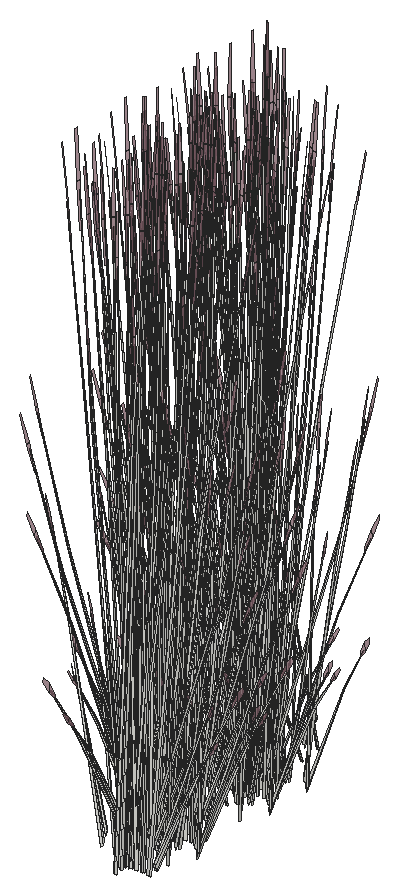
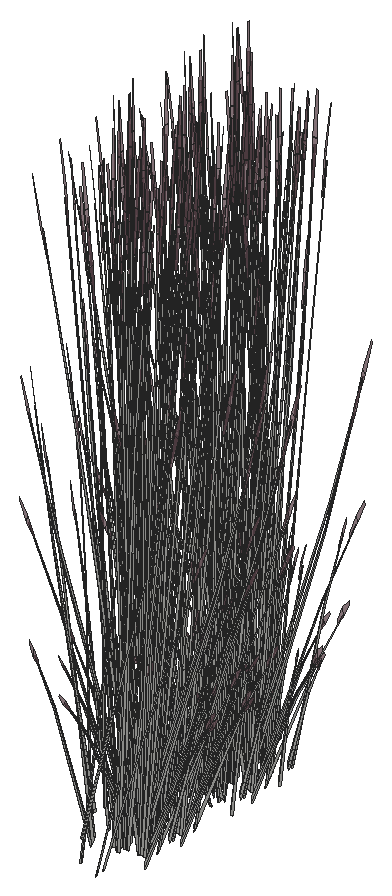
# SketchUp Ruby script. Lengths in inches.
U = 1.inch
M = Sketchup.active_model
def pt(a) = Geom::Point3d.new(a.map { |v| v * U })
def face(e, loops, mat)
  f = e.add_face(loops[0].map { |a| pt(a) })
  loops[1..].each { |l| e.add_face(l.map { |a| pt(a) }).erase! }
  f.material = f.back_material = mat if mat
  f
end
# faces: each face lists its corners as indices into pts; further lists are holes
def faces(e, pts, list, mat = nil) = list.each { |f| face(e, (f[0].is_a?(Array) ? f : [f]).map { |l| l.map { |i| pts[i] } }, mat) }
# xy, xz, yz: faces in a plane at the given z, y or x. An outline is a flat list of corners, or four numbers for a rectangle; further outlines are holes
def ring(l) = l.size == 4 ? [[l[0], l[1]], [l[2], l[1]], [l[2], l[3]], [l[0], l[3]]] : l.each_slice(2).to_a
def flat(e, list, mat, &to3) = list.each { |f| face(e, (f[0].is_a?(Array) ? f : [f]).map { |l| ring(l).map { |u, v| to3.(u, v) } }, mat) }
def xy(e, z, list, mat = nil) = flat(e, list, mat) { |x, y| [x, y, z] }
def xz(e, y, list, mat = nil) = flat(e, list, mat) { |x, z| [x, y, z] }
def yz(e, x, list, mat = nil) = flat(e, list, mat) { |y, z| [x, y, z] }
def lines(e, pts, list) = list.each { |a, b| e.add_line(pt(pts[a]), pt(pts[b])) }
# prism: a flat outline (further loops are holes) pulled along v
def prism(e, loops, v, mat = nil)
  f = face(e, loops, mat); d = Geom::Vector3d.new(v.map { |x| x * U })
  f.pushpull(f.normal.samedirection?(d) ? d.length : -d.length)
end
def box(e, o, s, mat = nil) = prism(e, [[o, [o[0] + s[0], o[1], o[2]], [o[0] + s[0], o[1] + s[1], o[2]], [o[0], o[1] + s[1], o[2]]]], [0, 0, s[2]], mat)
def at(x, y, z, deg = 0) = Geom::Transformation.translation(pt([x, y, z])) * Geom::Transformation.rotation(ORIGIN, Z_AXIS, deg.degrees)
def axes(o, x, y, z) = Geom::Transformation.new([*x, 0, *y, 0, *z, 0, *pt(o).to_a, 1])
def part(name) = M.definitions.add(name)
# library, detail: a bought-in or finely detailed component or shape, given as its bounding box
def library(name, o, s) = part(name).tap { |d| box(d.entities, o, s) }
def detail(e, o, s) = box(e.add_group.entities, o, s)
def put(e, d, t, mat = nil) = e.add_instance(d, t).tap { |i| i.material = mat if mat }
def group(e, t, mat = nil) = e.add_group.tap { |g| g.transformation = t; g.material = mat if mat }.entities
root = M.entities
M.materials.add("LightPink_Translucent").color = [144, 107, 117]
M.materials["LightPink_Translucent"].alpha = 0.75
c1 = part("blade")
p = [[2.15,0.21,22],[0,0.17,0],[0.09,0.45,0],[2.18,0.31,22],[2.29,0.31,22],[0.38,0.45,0],
  [2.48,0.24,33],[2.49,0.24,33],[2.48,0.22,33]]
faces(c1.entities,p,[[0,1,2,3],[4,5,2,3],[6,3,4,7],[8,0,3,6]])
c2 = part("seeds")
p = [[0.3,-0.1,1.38],[-0.01,-0.03,1.59],[-0.01,-0.03,0.03],[0.14,-0.07,-0.07],[0.29,-0.03,3],[0.15,0.01,3.11]]
faces(c2.entities,p,[[0,1,2,3],[1,0,4,5]],"LightPink_Translucent")
c3 = part("blade with seeds")
put(c3.entities,c1,at(0,0,0))
put(c3.entities,c2,axes([2.4,0.25,30.99],[1.5799,-0.05474,1.17369],[-0.12525,1.92788,0.29478],[-0.07173,-0.02425,1.56792]))
put(root,c3,axes([429.91,427.55,152.09],[-0.44036,0.12519,0.14904],[-0.10874,-0.46588,0.29641],[0.03927,0.06788,1.35512]))
put(root,c3,axes([427.96,431.05,152.34],[0.21377,0.16416,0.97034],[-0.31132,0.09868,0.71294],[-0.06661,-0.12616,0.21373]))
put(root,c3,axes([428.47,431.92,154.21],[-0.34944,-0.22798,-0.60019],[0.24834,-0.39949,0.07243],[-0.1266,-0.13612,0.84903]))
put(root,c3,axes([429.63,428.45,152.01],[-0.51796,-0.09937,0.41563],[0.10541,-0.56124,0.1631],[0.07569,0.05419,1.44303]))
put(root,c3,axes([429.21,429.83,151.86],[-0.13371,-0.40664,0],[0.38182,-0.1424,0],[0,0,1.30413]))
put(root,c3,axes([428.96,429.45,152.21],[-0.07906,0.42093,0.12232],[-0.38625,-0.07307,-0.3493],[-0.07029,-0.04322,1.07074]))
put(root,c3,axes([429.71,429.77,151.85],[0.43024,-0.16003,-0.16218],[0.15118,0.46099,0.00007],[0.04749,-0.01769,1.46908]))
put(root,c3,axes([429.86,429.97,152.09],[0.11838,-0.46875,0.14904],[0.43321,0.13265,0.29641],[-0.07483,0.00228,1.35512]))
put(root,c3,axes([429.77,428.9,151.87],[0.28606,0.30466,0],[-0.28606,0.30466,0],[0,0,1.42996]))
put(root,c3,axes([427.79,431.54,151.26],[-0.0397,0.06213,1.48974],[-0.40116,0.13396,-0.22758],[-0.09691,-0.12186,0.25375]))
put(root,c3,axes([430.54,428.77,152.09],[-0.32198,-0.34356,0.14904],[0.32447,-0.33323,0.29641],[-0.03556,0.07016,1.35512]))
put(root,c3,axes([431.83,429.09,152.34],[-0.2532,0.07787,0.97034],[0.11918,-0.32181,0.71294],[0.13432,0.02202,0.21373]))
put(root,c3,axes([430.7,431.77,151.26],[-0.06134,-0.03716,1.48974],[-0.15755,-0.41512,-0.22758],[0.10629,-0.11265,0.25375]))
put(root,c3,axes([429.12,430.02,151.86],[-0.41314,-0.21175,0],[0.19883,-0.43999,0],[0,0,1.37455]))
put(root,c3,axes([429.46,429.45,152.08],[-0.40016,-0.37963,-0.21282],[0.33672,-0.42629,0.46574],[-0.10776,0.04441,1.42109]))
put(root,c3,axes([428.41,430.18,152.09],[0.38354,0.23583,0.41945],[-0.22925,0.42288,0],[-0.08735,-0.05371,1.33059]))
put(root,c3,axes([429.76,428.55,152.3],[0.19883,-0.425,0.37796],[0.41314,0.20454,-0.1819],[0,0.09797,1.2135]))
put(root,c3,axes([429.68,428.79,151.9375],[0,0.54548,-0.04762],[-0.51243,0,0],[0,0.01714,1.5153]))
put(root,c3,axes([428.1875,430.43,152],[-0.25622,0.47263,0],[-0.42866,-0.26357,-0.43598],[-0.09763,-0.06003,1.38303]))
put(root,c3,axes([430.7,432.94,154.21],[0.21406,-0.37215,-0.60019],[0.37511,0.26448,0.07243],[0.12781,-0.13483,0.84903]))
put(root,c3,axes([428.38,431.86,152],[-0.25622,-0.47263,0],[0.42866,-0.26357,-0.43598],[0.09763,-0.06003,1.38303]))
put(root,c3,axes([430.8,428.78,152.09],[0,-0.47166,0.41945],[0.45849,0,0],[0,0.10742,1.33059]))
put(root,c3,axes([429.66,429.14,152.3],[0.44501,-0.02912,0.37796],[0.04024,0.48332,-0.1819],[-0.07967,0.04899,1.2135]))
put(root,c3,axes([429.93,428.64,152.21],[0.38182,-0.13755,0.12232],[0.13371,0.39278,-0.3493],[0,0.08644,1.07074]))
put(root,c3,axes([428.95,431.29,151.8],[-0.28319,0.27058,-0.03288],[-0.25948,-0.29635,-0.1491],[-0.01827,-0.08397,0.4918]))
put(root,c3,axes([431.35,429.6,152.1875],[-0.0987,-0.116,1.20808],[0.12841,-0.38374,-0.25981],[0.19968,0.05198,0.51652]))
put(root,c3,axes([429.59,430.02,151.86],[0.41314,0.21175,0],[-0.19883,0.43999,0],[0,0,1.47801]))
put(root,c3,axes([429.75,430.49,151.85],[-0.25302,-0.47428,-0.04344],[0.42866,-0.26357,0.43598],[-0.10563,0.04516,1.38235]))
put(root,c3,axes([431.01,432.6,152.1875],[-0.1464,-0.01397,1.20808],[-0.14998,-0.37477,-0.25981],[0.17985,-0.10602,0.51652]))
put(root,c3,axes([429.66,429.34,152.21],[0.30276,0.28338,0.12232],[-0.25254,0.31972,-0.3493],[-0.07029,0.04322,1.07074]))
put(root,c3,axes([431.18,431.91,152.34],[-0.1365,0.2401,0.97034],[-0.11733,-0.32258,0.71294],[0.11274,-0.08083,0.21373]))
put(root,c3,axes([430.45,429.83,154.21],[0.40965,0.01136,-0.60019],[-0.02751,0.47821,0.07243],[0.17355,0.05047,0.84903]))
put(root,c3,axes([429.99,430.22,152.09],[0.38354,-0.23583,0.41945],[0.22925,0.42288,0],[-0.08735,0.05371,1.33059]))
put(root,c3,axes([429.44,429.85,151.9375],[0.17817,0.54185,-0.05079],[-0.50909,0.18987,0],[0.00622,0.01892,1.45452]))
put(root,c3,axes([426.88,429.6,152.1875],[0.14242,0.03872,1.20808],[0.09179,0.39548,-0.25981],[-0.19345,0.07403,0.51652]))
put(root,c3,axes([428.89,433.16,152.25],[-0.04775,-0.53819,-0.2458],[0.49736,-0.03254,-0.42242],[0.08758,-0.07169,1.34921]))
put(root,c3,axes([431.12,428.86,152.01],[0.51243,0,0],[0,0.52715,-0.43598],[0,0.12006,1.38303]))
put(root,c3,axes([427.54,431.78,151.8],[-0.11822,0.38513,-0.03288],[-0.36385,-0.11847,-0.1491],[-0.05524,-0.06299,0.4918]))
put(root,c3,axes([428.66,433.73,152.25],[-0.46151,-0.22505,-0.2458],[0.22222,-0.475,-0.42242],[-0.0145,-0.11662,1.34921]))
put(root,c3,axes([430.91,429.14,151.86],[-0.51218,-0.00377,-0.04204],[0,-0.52715,0.42192],[-0.0161,0.12,1.33776]))
put(root,c3,axes([429.8,428.68,152.25],[0.46151,0.22505,-0.2458],[-0.22222,0.475,-0.42242],[0.0145,0.11662,1.34921]))
put(root,c3,axes([427.34,433.54,152],[-0.51243,0,0],[0,-0.52715,-0.43598],[0,-0.12006,1.38303]))
put(root,c3,axes([426.58,430.43,152.34],[0.17079,-0.21377,0.97034],[0.06739,0.33841,0.71294],[-0.12342,0.0606,0.21373]))
put(root,c3,axes([427.43,432.6,152.1875],[0.08001,0.13132,1.20808],[-0.18437,0.35694,-0.25981],[-0.18931,-0.08532,0.51652]))
put(root,c3,axes([429.57,429.24,152.25],[0.04775,0.53819,-0.2458],[-0.49736,0.03254,-0.42242],[-0.08758,0.07169,1.34921]))
put(root,c3,axes([427.76,432.48,154.21],[-0.40965,-0.01136,-0.60019],[0.02751,-0.47821,0.07243],[-0.17355,-0.05047,0.84903]))
put(root,c3,axes([429.76,430.25,151.97],[0.51304,0.1533,0.25983],[-0.12835,0.54797,-0.30828],[-0.08491,0.06858,1.39295]))
put(root,c3,axes([427.74,433.4,151.97],[-0.38118,0.39654,0.25983],[-0.38142,-0.39237,-0.30828],[-0.01331,-0.11261,1.39295]))
put(root,c3,axes([428.95,433.59,152.06],[0.46174,0.2286,0.2033],[-0.22222,0.475,0.42242],[0,-0.1095,1.35626]))
put(root,c3,axes([428.77,434.23,152.06],[0.10862,-0.55889,-0.19793],[0.515,0.09742,0.43313],[-0.08999,-0.07718,1.32161]))
put(root,c3,axes([430.42,430.2,152.34],[-0.23074,-0.13562,0.97034],[0.29794,-0.1378,0.71294],[0.08036,0.11673,0.21373]))
put(root,c3,axes([426.95,432.99,152.34],[0.26163,-0.03375,0.97034],[-0.16596,0.29737,0.71294],[-0.12929,-0.04461,0.21373]))
put(root,c3,axes([428.8,433.27,152.3],[-0.44501,0.02912,0.37796],[-0.04024,-0.48332,-0.1819],[0.07967,-0.04899,1.2135]))
put(root,c3,axes([427.65,433.62,152.09],[0,0.47166,0.41945],[-0.45849,0,0],[0,-0.10742,1.33059]))
put(root,c3,axes([430.08,430.55,152],[0.25622,0.47263,0],[-0.42866,0.26357,-0.43598],[-0.09763,0.06003,1.38303]))
put(root,c3,axes([430.27,431.98,152.01],[0.25622,-0.47263,0],[0.42866,0.26357,-0.43598],[0.09763,0.06003,1.38303]))
put(root,c3,axes([430.48,430.7,151.26],[0.02986,-0.06809,1.48974],[0.37589,-0.20055,-0.22758],[0.11396,0.1038,0.25375]))
put(root,c3,axes([429.86,428.67,152.4],[-0.01119,-0.44408,1.19347],[0.50665,0.11511,0.50532],[-0.11983,0.243,1.12654]))
put(root,c3,axes([428.79,433.44,151.99],[0.17817,0.52741,0.38653],[-0.50909,0.1834,0.15168],[0.00622,-0.09691,1.34202]))
put(root,c3,axes([427.03,430.65,151.26],[0.05497,0.04712,1.48974],[0.09321,0.43661,-0.22758],[-0.12183,0.0931,0.25375]))
put(root,c3,axes([431.28,433.85,151.67],[-0.26394,0.0566,1.1961],[-0.04201,-0.45055,0.06846],[0.18486,-0.06819,0.68062]))
put(root,c3,axes([431.76,433.45,151.91],[-0.25407,-0.3016,-0.05481],[0.27826,-0.27635,-0.2485],[0.07884,-0.01946,0.81966]))
put(root,c3,axes([428.7,433.86,152.3],[-0.19883,0.425,0.37796],[-0.41314,-0.20454,-0.1819],[0,-0.09797,1.2135]))
put(root,c3,axes([429.43,433.49,151.86],[0,-0.54574,0],[0.51243,0,0],[0,0,1.51605]))
put(root,c3,axes([430.46,430.82,152.25],[-0.26279,-0.01479,0.88755],[0.17355,-0.31417,0.49003],[0.10382,0.11162,0.6962]))
put(root,c3,axes([430.05,432.22,152.09],[-0.38354,-0.23583,0.41945],[0.22925,-0.42288,0],[0.08735,0.05371,1.33059]))
put(root,c3,axes([430.8,433.88,154.21],[0.3601,-0.20831,-0.60019],[0.20068,0.4288,0.07243],[0.17399,-0.04871,0.84903]))
put(root,c3,axes([429.18,433.14,151.99],[-0.33979,0.42804,0.38653],[-0.40368,-0.37784,0.15168],[0.08192,-0.04272,1.34202]))
put(root,c3,axes([429.56,433.91,151.94],[-0.38118,-0.40596,-0.0518],[0.38142,-0.40621,0],[-0.01331,-0.01418,1.48322]))
put(root,c3,axes([428.59,432.4375,152.09],[-0.11838,0.46875,0.14904],[-0.43321,-0.13265,0.29641],[0.07483,-0.00228,1.35512]))
put(root,c3,axes([428.42,432.82,151.35],[-0.40337,0.18883,1.08919],[-0.12839,-0.54182,0.42321],[0.24769,0.00901,1.23883]))
put(root,c3,axes([429.5,432.96,152.21],[0.07906,-0.42093,0.12232],[0.38625,0.07307,-0.3493],[0.07029,0.04322,1.07074]))
put(root,c3,axes([429.6,430.06,152.1875],[0.00723,-0.15635,1.20808],[0.34559,-0.17464,-0.25981],[0.10668,0.18713,0.51652]))
put(root,c3,axes([428.83,433.96,151.99],[0.51796,0.09937,0.38653],[-0.10541,0.56124,0.15168],[-0.07569,-0.05419,1.34202]))
put(root,c3,axes([431.57,433.55,151.26],[-0.02142,-0.07161,1.48974],[0.14855,-0.41887,-0.22758],[0.14984,-0.00603,0.25375]))
put(root,c3,axes([427.14,433.48,151.26],[0.01039,0.07433,1.48974],[-0.20952,0.38819,-0.22758],[-0.14882,-0.01957,0.25375]))
put(root,c3,axes([429.33,433.07,152.3],[-0.24618,-0.39589,0.37796],[0.37289,-0.27878,-0.1819],[0.07967,0.04899,1.2135]))
put(root,c3,axes([428.03,431.36,152.34],[-0.01061,-0.28045,0.97034],[0.26501,0.20003,0.71294],[-0.05212,0.13367,0.21373]))
put(root,c3,axes([428.55,434.85,152.09],[0.44036,-0.12519,0.14904],[0.10874,0.46588,0.29641],[-0.03927,-0.06788,1.35512]))
put(root,c3,axes([429.46,433.09,152.25],[0.41376,-0.31314,-0.2458],[0.27514,0.44246,-0.42242],[0.10209,0.04493,1.34921]))
put(root,c3,axes([428.73,430.6875,151.26],[0.06632,-0.02567,1.48974],[0.39894,0.14126,-0.22758],[0.01167,0.15921,0.25375]))
put(root,c3,axes([429.78,433.61,151.86],[0.45849,0,0],[0,0.4883,0],[0,0,1.50718]))
put(root,c3,axes([429,434.22,152.25],[-0.41376,0.31314,-0.2458],[-0.27514,-0.44246,-0.42242],[-0.10209,-0.04493,1.34921]))
put(root,c3,axes([429.91,432.46,152.09],[-0.44036,0.12519,0.14904],[-0.10874,-0.46588,0.29641],[0.03927,0.06788,1.35512]))
put(root,c3,axes([427.8125,430.75,152.38],[0.37228,-0.08352,0.05498],[0.08559,0.3365,-0.7291],[-0.0236,0.17034,0.65354]))
put(root,c3,axes([429.63,433.36,152.01],[-0.51796,-0.09937,0.41563],[0.10541,-0.56124,0.1631],[0.07569,0.05419,1.44303]))
put(root,c3,axes([429.21,434.74,151.86],[-0.13371,-0.40664,0],[0.38182,-0.1424,0],[0,0,1.30413]))
put(root,c3,axes([428.96,434.36,152.21],[-0.07906,0.42093,0.12232],[-0.38625,-0.07307,-0.3493],[-0.07029,-0.04322,1.07074]))
put(root,c3,axes([429.71,434.6875,151.85],[0.43024,-0.16003,-0.16218],[0.15118,0.46099,0.00007],[0.04749,-0.01769,1.46908]))
put(root,c3,axes([429.86,434.88,152.09],[0.11838,-0.46875,0.14904],[0.43321,0.13265,0.29641],[-0.07483,0.00228,1.35512]))
put(root,c3,axes([429.77,433.82,151.87],[0.28606,0.30466,0],[-0.28606,0.30466,0],[0,0,1.42996]))
put(root,c3,axes([430.54,433.68,152.09],[-0.32198,-0.34356,0.14904],[0.32447,-0.33323,0.29641],[-0.03556,0.07016,1.35512]))
put(root,c3,axes([431.83,434,152.34],[-0.2532,0.07787,0.97034],[0.11918,-0.32181,0.71294],[0.13432,0.02202,0.21373]))
put(root,c3,axes([428.85,430.51,154.21],[0.19559,0.38351,-0.60019],[-0.40262,0.21373,0.07243],[0.04574,0.1853,0.84903]))
put(root,c3,axes([429.12,434.93,151.86],[-0.41314,-0.21175,0],[0.19883,-0.43999,0],[0,0,1.37455]))
put(root,c3,axes([429.46,434.37,152.08],[-0.40016,-0.37963,-0.21282],[0.33672,-0.42629,0.46574],[-0.10776,0.04441,1.42109]))
put(root,c3,axes([428.41,435.09,152.09],[0.38354,0.23583,0.41945],[-0.22925,0.42288,0],[-0.08735,-0.05371,1.33059]))
put(root,c3,axes([427.72,431.11,152.1875],[0.12932,-0.07441,1.20808],[0.31929,0.22435,-0.25981],[-0.09503,0.19413,0.51652]))
put(root,c3,axes([429.76,433.46,152.3],[0.19883,-0.425,0.37796],[0.41314,0.20454,-0.1819],[0,0.09797,1.2135]))
put(root,c3,axes([429.68,433.7,151.9375],[0,0.54548,-0.04762],[-0.51243,0,0],[0,0.01714,1.5153]))
put(root,c3,axes([428.1875,435.34,152],[-0.25622,0.47263,0],[-0.42866,-0.26357,-0.43598],[-0.09763,-0.06003,1.38303]))
put(root,c3,axes([430.8,433.7,152.09],[0,-0.47166,0.41945],[0.45849,0,0],[0,0.10742,1.33059]))
put(root,c3,axes([429.66,434.05,152.3],[0.44501,-0.02912,0.37796],[0.04024,0.48332,-0.1819],[-0.07967,0.04899,1.2135]))
put(root,c3,axes([429.93,433.56,152.21],[0.38182,-0.13755,0.12232],[0.13371,0.39278,-0.3493],[0,0.08644,1.07074]))
put(root,c3,axes([429.88,438.73,152.1875],[-0.11649,0.09547,1.20808],[-0.34886,-0.1671,-0.25981],[0.06467,-0.20781,0.51652]))
put(root,c3,axes([429.35,439.0625,154.21],[-0.19559,-0.38351,-0.60019],[0.40262,-0.21373,0.07243],[-0.04574,-0.1853,0.84903]))
put(root,c3,axes([428.08,438.55,152.1875],[-0.02482,0.15429,1.20808],[-0.36278,0.12916,-0.25981],[-0.0848,-0.19943,0.51652]))
put(root,c3,axes([431.35,434.51,152.1875],[-0.0987,-0.116,1.20808],[0.12841,-0.38374,-0.25981],[0.19968,0.05198,0.51652]))
put(root,c3,axes([429.02,438.21,151.26],[-0.06874,0.01699,1.48974],[-0.38012,-0.19128,-0.22758],[0.00638,-0.15955,0.25375]))
put(root,c3,axes([429.59,434.9375,151.86],[0.41314,0.21175,0],[-0.19883,0.43999,0],[0,0,1.47801]))
put(root,c3,axes([430.17,439.4375,154.21],[0.01066,-0.43628,-0.60019],[0.44902,0.0293,0.07243],[0.04739,-0.18483,0.84903]))
put(root,c3,axes([429.75,435.41,151.85],[-0.25302,-0.47428,-0.04344],[0.42866,-0.26357,0.43598],[-0.10563,0.04516,1.38235]))
put(root,c3,axes([429.66,434.26,152.21],[0.30276,0.28338,0.12232],[-0.25254,0.31972,-0.3493],[-0.07029,0.04322,1.07074]))
put(root,c3,axes([430.45,434.75,154.21],[0.40965,0.01136,-0.60019],[-0.02751,0.47821,0.07243],[0.17355,0.05047,0.84903]))
put(root,c3,axes([429.46,437.97,152.34],[0.05257,0.27504,0.97034],[-0.29163,-0.15233,0.71294],[0.03138,-0.14083,0.21373]))
put(root,c3,axes([429.99,435.13,152.09],[0.38354,-0.23583,0.41945],[0.22925,0.42288,0],[-0.08735,0.05371,1.33059]))
put(root,c3,axes([429.44,434.76,151.9375],[0.17817,0.54185,-0.05079],[-0.50909,0.18987,0],[0.00622,0.01892,1.45452]))
put(root,c3,axes([426.88,434.51,152.1875],[0.14242,0.03872,1.20808],[0.09179,0.39548,-0.25981],[-0.19345,0.07403,0.51652]))
put(root,c3,axes([431.12,433.78,152.01],[0.51243,0,0],[0,0.52715,-0.43598],[0,0.12006,1.38303]))
put(root,c3,axes([430.91,434.05,151.86],[-0.51218,-0.00377,-0.04204],[0,-0.52715,0.42192],[-0.0161,0.12,1.33776]))
put(root,c3,axes([429.8,433.59,152.25],[0.46151,0.22505,-0.2458],[-0.22222,0.475,-0.42242],[0.0145,0.11662,1.34921]))
put(root,c3,axes([426.58,435.34,152.34],[0.17079,-0.21377,0.97034],[0.06739,0.33841,0.71294],[-0.12342,0.0606,0.21373]))
put(root,c3,axes([429.57,434.15,152.25],[0.04775,0.53819,-0.2458],[-0.49736,0.03254,-0.42242],[-0.08758,0.07169,1.34921]))
put(root,c3,axes([427.96,438.3,152.34],[0.21377,0.16416,0.97034],[-0.31132,0.09868,0.71294],[-0.06661,-0.12616,0.21373]))
put(root,c3,axes([428.47,439.17,154.21],[-0.34944,-0.22798,-0.60019],[0.24834,-0.39949,0.07243],[-0.1266,-0.13612,0.84903]))
put(root,c3,axes([427.79,438.8,151.26],[-0.0397,0.06213,1.48974],[-0.40116,0.13396,-0.22758],[-0.09691,-0.12186,0.25375]))
put(root,c3,axes([429.76,435.16,151.97],[0.51304,0.1533,0.25983],[-0.12835,0.54797,-0.30828],[-0.08491,0.06858,1.39295]))
put(root,c3,axes([430.7,439.03,151.26],[-0.06134,-0.03716,1.48974],[-0.15755,-0.41512,-0.22758],[0.10629,-0.11265,0.25375]))
put(root,c3,axes([430.42,435.11,152.34],[-0.23074,-0.13562,0.97034],[0.29794,-0.1378,0.71294],[0.08036,0.11673,0.21373]))
put(root,c3,axes([430.7,440.2,154.21],[0.21406,-0.37215,-0.60019],[0.37511,0.26448,0.07243],[0.12781,-0.13483,0.84903]))
put(root,c3,axes([430.08,435.46,152],[0.25622,0.47263,0],[-0.42866,0.26357,-0.43598],[-0.09763,0.06003,1.38303]))
put(root,c3,axes([428.38,439.11,152],[-0.25622,-0.47263,0],[0.42866,-0.26357,-0.43598],[0.09763,-0.06003,1.38303]))
put(root,c3,axes([428.95,438.54,151.8],[-0.28319,0.27058,-0.03288],[-0.25948,-0.29635,-0.1491],[-0.01827,-0.08397,0.4918]))
put(root,c3,axes([430.48,435.62,151.26],[0.02986,-0.06809,1.48974],[0.37589,-0.20055,-0.22758],[0.11396,0.1038,0.25375]))
put(root,c3,axes([429.86,433.59,152.4],[-0.01119,-0.44408,1.19347],[0.50665,0.11511,0.50532],[-0.11983,0.243,1.12654]))
put(root,c3,axes([427.03,435.56,151.26],[0.05497,0.04712,1.48974],[0.09321,0.43661,-0.22758],[-0.12183,0.0931,0.25375]))
put(root,c3,axes([430.46,435.73,152.25],[-0.26279,-0.01479,0.88755],[0.17355,-0.31417,0.49003],[0.10382,0.11162,0.6962]))
put(root,c3,axes([431.01,439.86,152.1875],[-0.1464,-0.01397,1.20808],[-0.14998,-0.37477,-0.25981],[0.17985,-0.10602,0.51652]))
put(root,c3,axes([431.18,439.17,152.34],[-0.1365,0.2401,0.97034],[-0.11733,-0.32258,0.71294],[0.11274,-0.08083,0.21373]))
put(root,c3,axes([429.6,434.97,152.1875],[0.00723,-0.15635,1.20808],[0.34559,-0.17464,-0.25981],[0.10668,0.18713,0.51652]))
put(root,c3,axes([428.03,436.27,152.34],[-0.01061,-0.28045,0.97034],[0.26501,0.20003,0.71294],[-0.05212,0.13367,0.21373]))
put(root,c3,axes([428.89,440.42,152.25],[-0.04775,-0.53819,-0.2458],[0.49736,-0.03254,-0.42242],[0.08758,-0.07169,1.34921]))
put(root,c3,axes([427.54,439.04,151.8],[-0.11822,0.38513,-0.03288],[-0.36385,-0.11847,-0.1491],[-0.05524,-0.06299,0.4918]))
put(root,c3,axes([428.66,440.98,152.25],[-0.46151,-0.22505,-0.2458],[0.22222,-0.475,-0.42242],[-0.0145,-0.11662,1.34921]))
put(root,c3,axes([428.73,435.6,151.26],[0.06632,-0.02567,1.48974],[0.39894,0.14126,-0.22758],[0.01167,0.15921,0.25375]))
put(root,c3,axes([427.34,440.79,152],[-0.51243,0,0],[0,-0.52715,-0.43598],[0,-0.12006,1.38303]))
put(root,c3,axes([427.43,439.85,152.1875],[0.08001,0.13132,1.20808],[-0.18437,0.35694,-0.25981],[-0.18931,-0.08532,0.51652]))
put(root,c3,axes([427.8125,435.67,152.38],[0.37228,-0.08352,0.05498],[0.08559,0.3365,-0.7291],[-0.0236,0.17034,0.65354]))
put(root,c3,axes([427.76,439.74,154.21],[-0.40965,-0.01136,-0.60019],[0.02751,-0.47821,0.07243],[-0.17355,-0.05047,0.84903]))
put(root,c3,axes([429.88,442.42,152.1875],[-0.11649,0.09547,1.20808],[-0.34886,-0.1671,-0.25981],[0.06467,-0.20781,0.51652]))
put(root,c3,axes([429.35,442.76,154.21],[-0.19559,-0.38351,-0.60019],[0.40262,-0.21373,0.07243],[-0.04574,-0.1853,0.84903]))
put(root,c3,axes([428.08,442.24,152.1875],[-0.02482,0.15429,1.20808],[-0.36278,0.12916,-0.25981],[-0.0848,-0.19943,0.51652]))
put(root,c3,axes([429.02,441.9,151.26],[-0.06874,0.01699,1.48974],[-0.38012,-0.19128,-0.22758],[0.00638,-0.15955,0.25375]))
put(root,c3,axes([427.74,440.66,151.97],[-0.38118,0.39654,0.25983],[-0.38142,-0.39237,-0.30828],[-0.01331,-0.11261,1.39295]))
put(root,c3,axes([430.17,443.13,154.21],[0.01066,-0.43628,-0.60019],[0.44902,0.0293,0.07243],[0.04739,-0.18483,0.84903]))
put(root,c3,axes([428.95,440.84,152.06],[0.46174,0.2286,0.2033],[-0.22222,0.475,0.42242],[0,-0.1095,1.35626]))
put(root,c3,axes([428.77,441.48,152.06],[0.10862,-0.55889,-0.19793],[0.515,0.09742,0.43313],[-0.08999,-0.07718,1.32161]))
put(root,c3,axes([428.85,435.42,154.21],[0.19559,0.38351,-0.60019],[-0.40262,0.21373,0.07243],[0.04574,0.1853,0.84903]))
put(root,c3,axes([426.95,440.25,152.34],[0.26163,-0.03375,0.97034],[-0.16596,0.29737,0.71294],[-0.12929,-0.04461,0.21373]))
put(root,c3,axes([427.72,436.02,152.1875],[0.12932,-0.07441,1.20808],[0.31929,0.22435,-0.25981],[-0.09503,0.19413,0.51652]))
put(root,c3,axes([429.46,441.66,152.34],[0.05257,0.27504,0.97034],[-0.29163,-0.15233,0.71294],[0.03138,-0.14083,0.21373]))
put(root,c3,axes([428.8,440.52,152.3],[-0.44501,0.02912,0.37796],[-0.04024,-0.48332,-0.1819],[0.07967,-0.04899,1.2135]))
put(root,c3,axes([427.65,440.875,152.09],[0,0.47166,0.41945],[-0.45849,0,0],[0,-0.10742,1.33059]))
put(root,c3,axes([430.27,439.23,152.01],[0.25622,-0.47263,0],[0.42866,0.26357,-0.43598],[0.09763,0.06003,1.38303]))
put(root,c3,axes([428.79,440.7,151.99],[0.17817,0.52741,0.38653],[-0.50909,0.1834,0.15168],[0.00622,-0.09691,1.34202]))
put(root,c3,axes([431.28,441.1,151.67],[-0.26394,0.0566,1.1961],[-0.04201,-0.45055,0.06846],[0.18486,-0.06819,0.68062]))
put(root,c3,axes([431.76,440.7,151.91],[-0.25407,-0.3016,-0.05481],[0.27826,-0.27635,-0.2485],[0.07884,-0.01946,0.81966]))
put(root,c3,axes([428.7,441.11,152.3],[-0.19883,0.425,0.37796],[-0.41314,-0.20454,-0.1819],[0,-0.09797,1.2135]))
put(root,c3,axes([429.43,440.74,151.86],[0,-0.54574,0],[0.51243,0,0],[0,0,1.51605]))
put(root,c3,axes([427.96,441.99,152.34],[0.21377,0.16416,0.97034],[-0.31132,0.09868,0.71294],[-0.06661,-0.12616,0.21373]))
put(root,c3,axes([428.47,442.86,154.21],[-0.34944,-0.22798,-0.60019],[0.24834,-0.39949,0.07243],[-0.1266,-0.13612,0.84903]))
put(root,c3,axes([430.05,439.48,152.09],[-0.38354,-0.23583,0.41945],[0.22925,-0.42288,0],[0.08735,0.05371,1.33059]))
put(root,c3,axes([430.8,441.14,154.21],[0.3601,-0.20831,-0.60019],[0.20068,0.4288,0.07243],[0.17399,-0.04871,0.84903]))
put(root,c3,axes([429.18,440.4,151.99],[-0.33979,0.42804,0.38653],[-0.40368,-0.37784,0.15168],[0.08192,-0.04272,1.34202]))
put(root,c3,axes([429.56,441.16,151.94],[-0.38118,-0.40596,-0.0518],[0.38142,-0.40621,0],[-0.01331,-0.01418,1.48322]))
put(root,c3,axes([428.59,439.69,152.09],[-0.11838,0.46875,0.14904],[-0.43321,-0.13265,0.29641],[0.07483,-0.00228,1.35512]))
put(root,c3,axes([428.42,440.07,151.35],[-0.40337,0.18883,1.08919],[-0.12839,-0.54182,0.42321],[0.24769,0.00901,1.23883]))
put(root,c3,axes([427.79,442.49,151.26],[-0.0397,0.06213,1.48974],[-0.40116,0.13396,-0.22758],[-0.09691,-0.12186,0.25375]))
put(root,c3,axes([429.5,440.21,152.21],[0.07906,-0.42093,0.12232],[0.38625,0.07307,-0.3493],[0.07029,0.04322,1.07074]))
put(root,c3,axes([428.83,441.21,151.99],[0.51796,0.09937,0.38653],[-0.10541,0.56124,0.15168],[-0.07569,-0.05419,1.34202]))
put(root,c3,axes([431.57,440.81,151.26],[-0.02142,-0.07161,1.48974],[0.14855,-0.41887,-0.22758],[0.14984,-0.00603,0.25375]))
put(root,c3,axes([430.7,442.72,151.26],[-0.06134,-0.03716,1.48974],[-0.15755,-0.41512,-0.22758],[0.10629,-0.11265,0.25375]))
put(root,c3,axes([427.14,440.73,151.26],[0.01039,0.07433,1.48974],[-0.20952,0.38819,-0.22758],[-0.14882,-0.01957,0.25375]))
put(root,c3,axes([429.33,440.32,152.3],[-0.24618,-0.39589,0.37796],[0.37289,-0.27878,-0.1819],[0.07967,0.04899,1.2135]))
put(root,c3,axes([428.55,442.11,152.09],[0.44036,-0.12519,0.14904],[0.10874,0.46588,0.29641],[-0.03927,-0.06788,1.35512]))
put(root,c3,axes([429.46,440.35,152.25],[0.41376,-0.31314,-0.2458],[0.27514,0.44246,-0.42242],[0.10209,0.04493,1.34921]))
put(root,c3,axes([429.78,440.86,151.86],[0.45849,0,0],[0,0.4883,0],[0,0,1.50718]))
put(root,c3,axes([430.7,443.89,154.21],[0.21406,-0.37215,-0.60019],[0.37511,0.26448,0.07243],[0.12781,-0.13483,0.84903]))
put(root,c3,axes([428.38,442.81,152],[-0.25622,-0.47263,0],[0.42866,-0.26357,-0.43598],[0.09763,-0.06003,1.38303]))
put(root,c3,axes([429,441.48,152.25],[-0.41376,0.31314,-0.2458],[-0.27514,-0.44246,-0.42242],[-0.10209,-0.04493,1.34921]))
put(root,c3,axes([429.91,439.72,152.09],[-0.44036,0.12519,0.14904],[-0.10874,-0.46588,0.29641],[0.03927,0.06788,1.35512]))
put(root,c3,axes([428.95,442.24,151.8],[-0.28319,0.27058,-0.03288],[-0.25948,-0.29635,-0.1491],[-0.01827,-0.08397,0.4918]))
put(root,c3,axes([429.63,440.61,152.01],[-0.51796,-0.09937,0.41563],[0.10541,-0.56124,0.1631],[0.07569,0.05419,1.44303]))
put(root,c3,axes([429.21,442,151.86],[-0.13371,-0.40664,0],[0.38182,-0.1424,0],[0,0,1.30413]))
put(root,c3,axes([428.96,441.61,152.21],[-0.07906,0.42093,0.12232],[-0.38625,-0.07307,-0.3493],[-0.07029,-0.04322,1.07074]))
put(root,c3,axes([429.71,441.94,151.85],[0.43024,-0.16003,-0.16218],[0.15118,0.46099,0.00007],[0.04749,-0.01769,1.46908]))
put(root,c3,axes([429.86,442.14,152.09],[0.11838,-0.46875,0.14904],[0.43321,0.13265,0.29641],[-0.07483,0.00228,1.35512]))
put(root,c3,axes([431.01,443.55,152.1875],[-0.1464,-0.01397,1.20808],[-0.14998,-0.37477,-0.25981],[0.17985,-0.10602,0.51652]))
put(root,c3,axes([429.77,441.07,151.87],[0.28606,0.30466,0],[-0.28606,0.30466,0],[0,0,1.42996]))
put(root,c3,axes([430.54,440.94,152.09],[-0.32198,-0.34356,0.14904],[0.32447,-0.33323,0.29641],[-0.03556,0.07016,1.35512]))
put(root,c3,axes([431.18,442.86,152.34],[-0.1365,0.2401,0.97034],[-0.11733,-0.32258,0.71294],[0.11274,-0.08083,0.21373]))
put(root,c3,axes([431.83,441.25,152.34],[-0.2532,0.07787,0.97034],[0.11918,-0.32181,0.71294],[0.13432,0.02202,0.21373]))
put(root,c3,axes([429.12,442.18,151.86],[-0.41314,-0.21175,0],[0.19883,-0.43999,0],[0,0,1.37455]))
put(root,c3,axes([429.46,441.62,152.08],[-0.40016,-0.37963,-0.21282],[0.33672,-0.42629,0.46574],[-0.10776,0.04441,1.42109]))
put(root,c3,axes([428.41,442.35,152.09],[0.38354,0.23583,0.41945],[-0.22925,0.42288,0],[-0.08735,-0.05371,1.33059]))
put(root,c3,axes([429.76,440.72,152.3],[0.19883,-0.425,0.37796],[0.41314,0.20454,-0.1819],[0,0.09797,1.2135]))
put(root,c3,axes([428.89,444.11,152.25],[-0.04775,-0.53819,-0.2458],[0.49736,-0.03254,-0.42242],[0.08758,-0.07169,1.34921]))
put(root,c3,axes([429.68,440.96,151.9375],[0,0.54548,-0.04762],[-0.51243,0,0],[0,0.01714,1.5153]))
put(root,c3,axes([427.54,442.73,151.8],[-0.11822,0.38513,-0.03288],[-0.36385,-0.11847,-0.1491],[-0.05524,-0.06299,0.4918]))
put(root,c3,axes([428.1875,442.59,152],[-0.25622,0.47263,0],[-0.42866,-0.26357,-0.43598],[-0.09763,-0.06003,1.38303]))
put(root,c3,axes([428.66,444.67,152.25],[-0.46151,-0.22505,-0.2458],[0.22222,-0.475,-0.42242],[-0.0145,-0.11662,1.34921]))
put(root,c3,axes([427.34,444.49,152],[-0.51243,0,0],[0,-0.52715,-0.43598],[0,-0.12006,1.38303]))
put(root,c3,axes([430.8,440.95,152.09],[0,-0.47166,0.41945],[0.45849,0,0],[0,0.10742,1.33059]))
put(root,c3,axes([429.66,441.31,152.3],[0.44501,-0.02912,0.37796],[0.04024,0.48332,-0.1819],[-0.07967,0.04899,1.2135]))
put(root,c3,axes([429.93,440.8125,152.21],[0.38182,-0.13755,0.12232],[0.13371,0.39278,-0.3493],[0,0.08644,1.07074]))
put(root,c3,axes([427.43,443.54,152.1875],[0.08001,0.13132,1.20808],[-0.18437,0.35694,-0.25981],[-0.18931,-0.08532,0.51652]))
put(root,c3,axes([427.76,443.43,154.21],[-0.40965,-0.01136,-0.60019],[0.02751,-0.47821,0.07243],[-0.17355,-0.05047,0.84903]))
put(root,c3,axes([431.35,441.77,152.1875],[-0.0987,-0.116,1.20808],[0.12841,-0.38374,-0.25981],[0.19968,0.05198,0.51652]))
put(root,c3,axes([429.59,442.19,151.86],[0.41314,0.21175,0],[-0.19883,0.43999,0],[0,0,1.47801]))
put(root,c3,axes([429.75,442.66,151.85],[-0.25302,-0.47428,-0.04344],[0.42866,-0.26357,0.43598],[-0.10563,0.04516,1.38235]))
put(root,c3,axes([429.66,441.51,152.21],[0.30276,0.28338,0.12232],[-0.25254,0.31972,-0.3493],[-0.07029,0.04322,1.07074]))
put(root,c3,axes([427.74,444.35,151.97],[-0.38118,0.39654,0.25983],[-0.38142,-0.39237,-0.30828],[-0.01331,-0.11261,1.39295]))
put(root,c3,axes([428.95,444.53,152.06],[0.46174,0.2286,0.2033],[-0.22222,0.475,0.42242],[0,-0.1095,1.35626]))
put(root,c3,axes([428.77,445.17,152.06],[0.10862,-0.55889,-0.19793],[0.515,0.09742,0.43313],[-0.08999,-0.07718,1.32161]))
put(root,c3,axes([430.45,442,154.21],[0.40965,0.01136,-0.60019],[-0.02751,0.47821,0.07243],[0.17355,0.05047,0.84903]))
put(root,c3,axes([429.99,442.39,152.09],[0.38354,-0.23583,0.41945],[0.22925,0.42288,0],[-0.08735,0.05371,1.33059]))
put(root,c3,axes([426.95,443.9375,152.34],[0.26163,-0.03375,0.97034],[-0.16596,0.29737,0.71294],[-0.12929,-0.04461,0.21373]))
put(root,c3,axes([429.44,442.01,151.9375],[0.17817,0.54185,-0.05079],[-0.50909,0.18987,0],[0.00622,0.01892,1.45452]))
put(root,c3,axes([426.88,441.77,152.1875],[0.14242,0.03872,1.20808],[0.09179,0.39548,-0.25981],[-0.19345,0.07403,0.51652]))
put(root,c3,axes([428.8,444.21,152.3],[-0.44501,0.02912,0.37796],[-0.04024,-0.48332,-0.1819],[0.07967,-0.04899,1.2135]))
put(root,c3,axes([427.65,444.57,152.09],[0,0.47166,0.41945],[-0.45849,0,0],[0,-0.10742,1.33059]))
put(root,c3,axes([431.12,441.03,152.01],[0.51243,0,0],[0,0.52715,-0.43598],[0,0.12006,1.38303]))
put(root,c3,axes([430.91,441.3,151.86],[-0.51218,-0.00377,-0.04204],[0,-0.52715,0.42192],[-0.0161,0.12,1.33776]))
put(root,c3,axes([429.8,440.85,152.25],[0.46151,0.22505,-0.2458],[-0.22222,0.475,-0.42242],[0.0145,0.11662,1.34921]))
put(root,c3,axes([430.27,442.92,152.01],[0.25622,-0.47263,0],[0.42866,0.26357,-0.43598],[0.09763,0.06003,1.38303]))
put(root,c3,axes([428.79,444.39,151.99],[0.17817,0.52741,0.38653],[-0.50909,0.1834,0.15168],[0.00622,-0.09691,1.34202]))
put(root,c3,axes([426.58,442.6,152.34],[0.17079,-0.21377,0.97034],[0.06739,0.33841,0.71294],[-0.12342,0.0606,0.21373]))
put(root,c3,axes([429.57,441.41,152.25],[0.04775,0.53819,-0.2458],[-0.49736,0.03254,-0.42242],[-0.08758,0.07169,1.34921]))
put(root,c3,axes([431.28,444.79,151.67],[-0.26394,0.0566,1.1961],[-0.04201,-0.45055,0.06846],[0.18486,-0.06819,0.68062]))
put(root,c3,axes([431.76,444.39,151.91],[-0.25407,-0.3016,-0.05481],[0.27826,-0.27635,-0.2485],[0.07884,-0.01946,0.81966]))
put(root,c3,axes([428.7,444.8,152.3],[-0.19883,0.425,0.37796],[-0.41314,-0.20454,-0.1819],[0,-0.09797,1.2135]))
put(root,c3,axes([429.43,444.43,151.86],[0,-0.54574,0],[0.51243,0,0],[0,0,1.51605]))
put(root,c3,axes([430.05,443.17,152.09],[-0.38354,-0.23583,0.41945],[0.22925,-0.42288,0],[0.08735,0.05371,1.33059]))
put(root,c3,axes([430.8,444.83,154.21],[0.3601,-0.20831,-0.60019],[0.20068,0.4288,0.07243],[0.17399,-0.04871,0.84903]))
put(root,c3,axes([429.18,444.09,151.99],[-0.33979,0.42804,0.38653],[-0.40368,-0.37784,0.15168],[0.08192,-0.04272,1.34202]))
put(root,c3,axes([429.56,444.86,151.94],[-0.38118,-0.40596,-0.0518],[0.38142,-0.40621,0],[-0.01331,-0.01418,1.48322]))
put(root,c3,axes([428.59,443.38,152.09],[-0.11838,0.46875,0.14904],[-0.43321,-0.13265,0.29641],[0.07483,-0.00228,1.35512]))
put(root,c3,axes([429.76,442.42,151.97],[0.51304,0.1533,0.25983],[-0.12835,0.54797,-0.30828],[-0.08491,0.06858,1.39295]))
put(root,c3,axes([428.42,443.76,151.35],[-0.40337,0.18883,1.08919],[-0.12839,-0.54182,0.42321],[0.24769,0.00901,1.23883]))
put(root,c3,axes([429.5,443.9,152.21],[0.07906,-0.42093,0.12232],[0.38625,0.07307,-0.3493],[0.07029,0.04322,1.07074]))
put(root,c3,axes([428.83,444.9,151.99],[0.51796,0.09937,0.38653],[-0.10541,0.56124,0.15168],[-0.07569,-0.05419,1.34202]))
put(root,c3,axes([429.88,447.85,152.1875],[-0.11649,0.09547,1.20808],[-0.34886,-0.1671,-0.25981],[0.06467,-0.20781,0.51652]))
put(root,c3,axes([431.57,444.5,151.26],[-0.02142,-0.07161,1.48974],[0.14855,-0.41887,-0.22758],[0.14984,-0.00603,0.25375]))
put(root,c3,axes([429.35,448.18,154.21],[-0.19559,-0.38351,-0.60019],[0.40262,-0.21373,0.07243],[-0.04574,-0.1853,0.84903]))
put(root,c3,axes([427.14,444.42,151.26],[0.01039,0.07433,1.48974],[-0.20952,0.38819,-0.22758],[-0.14882,-0.01957,0.25375]))
put(root,c3,axes([430.42,442.37,152.34],[-0.23074,-0.13562,0.97034],[0.29794,-0.1378,0.71294],[0.08036,0.11673,0.21373]))
put(root,c3,axes([429.33,444.02,152.3],[-0.24618,-0.39589,0.37796],[0.37289,-0.27878,-0.1819],[0.07967,0.04899,1.2135]))
put(root,c3,axes([428.08,447.66,152.1875],[-0.02482,0.15429,1.20808],[-0.36278,0.12916,-0.25981],[-0.0848,-0.19943,0.51652]))
put(root,c3,axes([429.02,447.33,151.26],[-0.06874,0.01699,1.48974],[-0.38012,-0.19128,-0.22758],[0.00638,-0.15955,0.25375]))
